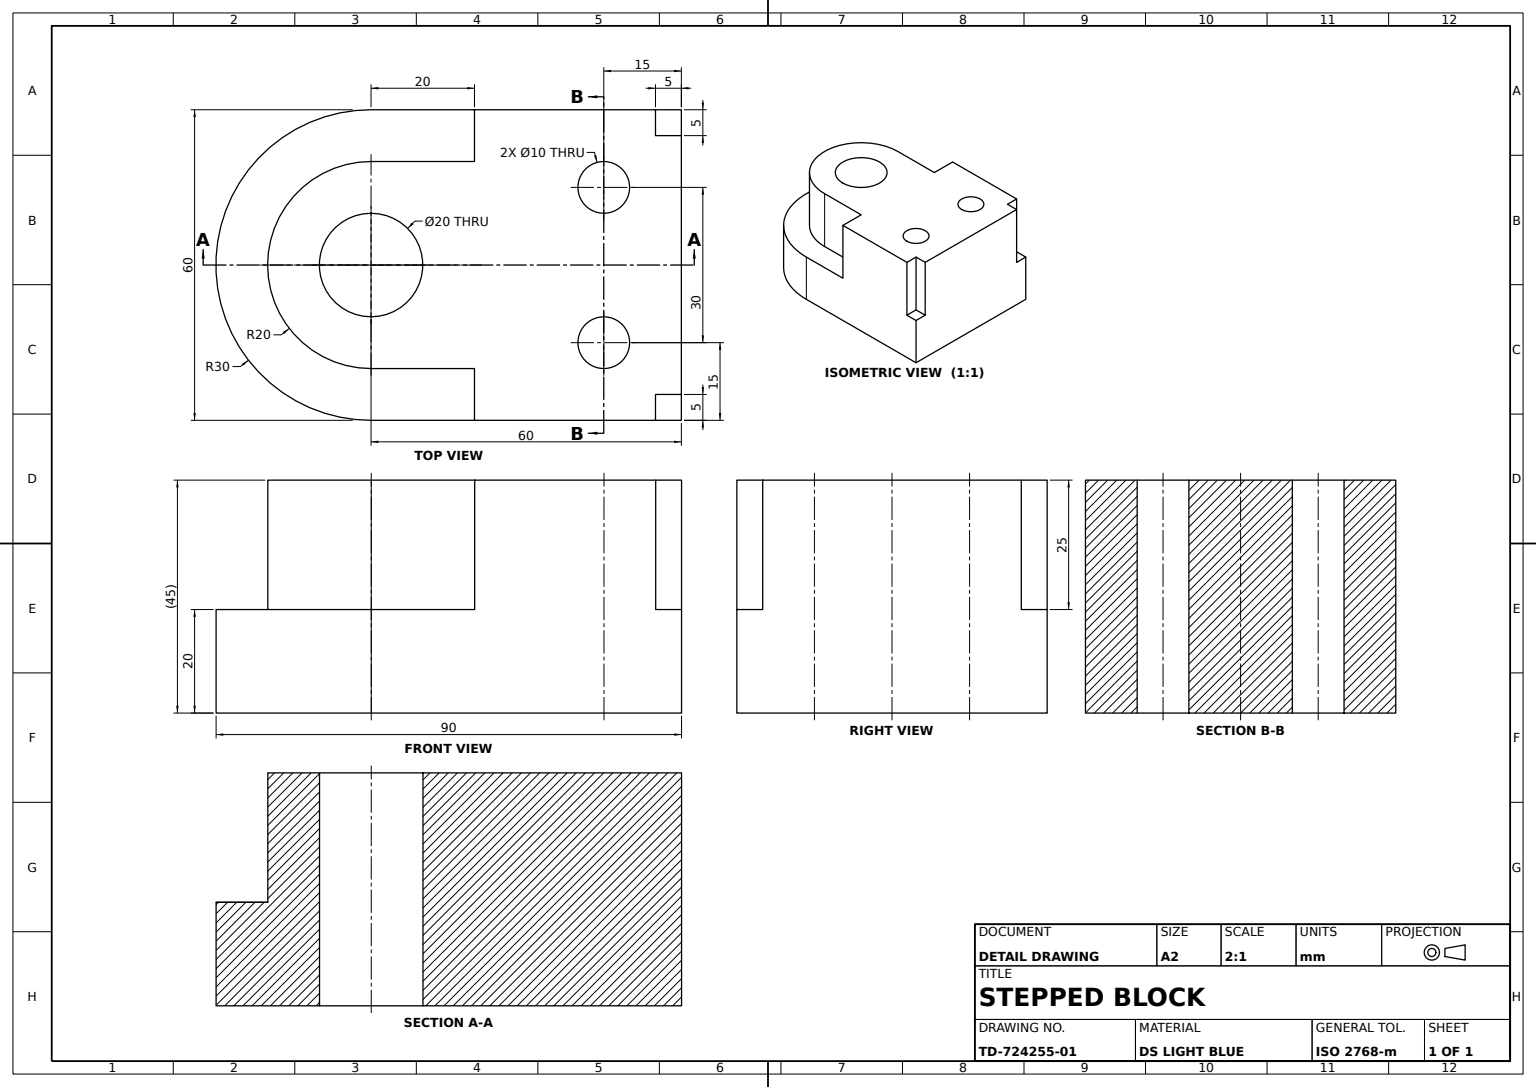
ISO-10303-21;
HEADER;
FILE_DESCRIPTION((''),'2;1');
FILE_NAME('','',(''),(''),'','','');
FILE_SCHEMA(('AUTOMOTIVE_DESIGN'));
ENDSEC;
DATA;
#1=APPLICATION_CONTEXT('');
#2=PRODUCT_CONTEXT('',#1,'mechanical');
#3=PRODUCT('','','',(#2));
#4=PRODUCT_DEFINITION_FORMATION('','',#3);
#5=PRODUCT_DEFINITION_CONTEXT('',#1,'design');
#6=PRODUCT_DEFINITION('','',#4,#5);
#7=PRODUCT_DEFINITION_SHAPE('','',#6);
#8=(LENGTH_UNIT()NAMED_UNIT(*)SI_UNIT(.MILLI.,.METRE.));
#9=(NAMED_UNIT(*)PLANE_ANGLE_UNIT()SI_UNIT($,.RADIAN.));
#10=(NAMED_UNIT(*)SI_UNIT($,.STERADIAN.)SOLID_ANGLE_UNIT());
#11=UNCERTAINTY_MEASURE_WITH_UNIT(LENGTH_MEASURE(0.005),#8,'distance_accuracy_value','');
#12=(GEOMETRIC_REPRESENTATION_CONTEXT(3)GLOBAL_UNCERTAINTY_ASSIGNED_CONTEXT((#11))GLOBAL_UNIT_ASSIGNED_CONTEXT((#8,#9,#10))REPRESENTATION_CONTEXT('',''));
#13=CARTESIAN_POINT('',(-30.,-30.,20.));
#14=VERTEX_POINT('',#13);
#15=CARTESIAN_POINT('',(30.,-30.,20.));
#16=VERTEX_POINT('',#15);
#17=CARTESIAN_POINT('',(0.,-30.,20.));
#18=DIRECTION('',(0.,0.,1.));
#19=DIRECTION('',(1.,0.,0.));
#20=AXIS2_PLACEMENT_3D('',#17,#18,#19);
#21=CIRCLE('',#20,30.);
#22=EDGE_CURVE('',#14,#16,#21,.T.);
#23=ORIENTED_EDGE('',*,*,#22,.F.);
#24=CARTESIAN_POINT('',(-30.,-30.,0.));
#25=VERTEX_POINT('',#24);
#26=CARTESIAN_POINT('',(-30.,-30.,10.));
#27=VECTOR('',#18,1000.);
#28=LINE('',#26,#27);
#29=EDGE_CURVE('',#25,#14,#28,.T.);
#30=ORIENTED_EDGE('',*,*,#29,.F.);
#31=CARTESIAN_POINT('',(30.,-30.,0.));
#32=VERTEX_POINT('',#31);
#33=CARTESIAN_POINT('',(0.,-30.,0.));
#34=AXIS2_PLACEMENT_3D('',#33,#18,#19);
#35=CIRCLE('',#34,30.);
#36=EDGE_CURVE('',#25,#32,#35,.T.);
#37=ORIENTED_EDGE('',*,*,#36,.T.);
#38=CARTESIAN_POINT('',(30.,-30.,10.));
#39=LINE('',#38,#27);
#40=EDGE_CURVE('',#32,#16,#39,.T.);
#41=ORIENTED_EDGE('',*,*,#40,.T.);
#42=EDGE_LOOP('',(#23,#30,#37,#41));
#43=FACE_BOUND('',#42,.T.);
#44=CARTESIAN_POINT('',(0.,-30.,10.));
#45=DIRECTION('',(0.,1.,0.));
#46=AXIS2_PLACEMENT_3D('',#44,#18,#45);
#47=CYLINDRICAL_SURFACE('',#46,30.);
#48=ADVANCED_FACE('',(#43),#47,.T.);
#49=CARTESIAN_POINT('',(20.,15.,45.));
#50=VERTEX_POINT('',#49);
#51=CARTESIAN_POINT('',(15.,15.,45.));
#52=AXIS2_PLACEMENT_3D('',#51,#18,#19);
#53=CIRCLE('',#52,5.);
#54=EDGE_CURVE('',#50,#50,#53,.T.);
#55=ORIENTED_EDGE('',*,*,#54,.T.);
#56=EDGE_LOOP('',(#55));
#57=FACE_BOUND('',#56,.T.);
#58=CARTESIAN_POINT('',(20.,15.,0.));
#59=VERTEX_POINT('',#58);
#60=CARTESIAN_POINT('',(15.,15.,0.));
#61=AXIS2_PLACEMENT_3D('',#60,#18,#19);
#62=CIRCLE('',#61,5.);
#63=EDGE_CURVE('',#59,#59,#62,.T.);
#64=ORIENTED_EDGE('',*,*,#63,.F.);
#65=EDGE_LOOP('',(#64));
#66=FACE_BOUND('',#65,.T.);
#67=CARTESIAN_POINT('',(15.,15.,21.84));
#68=AXIS2_PLACEMENT_3D('',#67,#18,#45);
#69=CYLINDRICAL_SURFACE('',#68,5.);
#70=ADVANCED_FACE('',(#57,#66),#69,.F.);
#71=CARTESIAN_POINT('',(-30.,-10.,20.));
#72=VERTEX_POINT('',#71);
#73=CARTESIAN_POINT('',(-30.,-10.,45.));
#74=VERTEX_POINT('',#73);
#75=CARTESIAN_POINT('',(-30.,-10.,0.));
#76=LINE('',#75,#27);
#77=EDGE_CURVE('',#72,#74,#76,.T.);
#78=ORIENTED_EDGE('',*,*,#77,.F.);
#79=CARTESIAN_POINT('',(-20.,-10.,20.));
#80=VERTEX_POINT('',#79);
#81=CARTESIAN_POINT('',(0.,-10.,20.));
#82=DIRECTION('',(-1.,0.,0.));
#83=VECTOR('',#82,1000.);
#84=LINE('',#81,#83);
#85=EDGE_CURVE('',#80,#72,#84,.T.);
#86=ORIENTED_EDGE('',*,*,#85,.F.);
#87=CARTESIAN_POINT('',(-20.,-10.,45.));
#88=VERTEX_POINT('',#87);
#89=LINE('',#79,#27);
#90=EDGE_CURVE('',#80,#88,#89,.T.);
#91=ORIENTED_EDGE('',*,*,#90,.T.);
#92=CARTESIAN_POINT('',(0.,-10.,45.));
#93=LINE('',#92,#83);
#94=EDGE_CURVE('',#88,#74,#93,.T.);
#95=ORIENTED_EDGE('',*,*,#94,.T.);
#96=EDGE_LOOP('',(#78,#86,#91,#95));
#97=FACE_BOUND('',#96,.T.);
#98=CARTESIAN_POINT('',(30.,-10.,20.));
#99=AXIS2_PLACEMENT_3D('',#98,#45,#82);
#100=PLANE('',#99);
#101=ADVANCED_FACE('',(#97),#100,.F.);
#102=CARTESIAN_POINT('',(-30.,30.,0.));
#103=VERTEX_POINT('',#102);
#104=CARTESIAN_POINT('',(30.,30.,0.));
#105=VERTEX_POINT('',#104);
#106=CARTESIAN_POINT('',(0.,30.,0.));
#107=VECTOR('',#19,1000.);
#108=LINE('',#106,#107);
#109=EDGE_CURVE('',#103,#105,#108,.T.);
#110=ORIENTED_EDGE('',*,*,#109,.T.);
#111=CARTESIAN_POINT('',(30.,0.,0.));
#112=DIRECTION('',(0.,-1.,0.));
#113=VECTOR('',#112,1000.);
#114=LINE('',#111,#113);
#115=EDGE_CURVE('',#105,#32,#114,.T.);
#116=ORIENTED_EDGE('',*,*,#115,.T.);
#117=ORIENTED_EDGE('',*,*,#36,.F.);
#118=CARTESIAN_POINT('',(-30.,0.,0.));
#119=VECTOR('',#45,1000.);
#120=LINE('',#118,#119);
#121=EDGE_CURVE('',#25,#103,#120,.T.);
#122=ORIENTED_EDGE('',*,*,#121,.T.);
#123=EDGE_LOOP('',(#110,#116,#117,#122));
#124=FACE_BOUND('',#123,.T.);
#125=ORIENTED_EDGE('',*,*,#63,.T.);
#126=EDGE_LOOP('',(#125));
#127=FACE_BOUND('',#126,.T.);
#128=CARTESIAN_POINT('',(-10.,15.,0.));
#129=VERTEX_POINT('',#128);
#130=CARTESIAN_POINT('',(-15.,15.,0.));
#131=AXIS2_PLACEMENT_3D('',#130,#18,#19);
#132=CIRCLE('',#131,5.);
#133=EDGE_CURVE('',#129,#129,#132,.T.);
#134=ORIENTED_EDGE('',*,*,#133,.T.);
#135=EDGE_LOOP('',(#134));
#136=FACE_BOUND('',#135,.T.);
#137=CARTESIAN_POINT('',(10.,-30.,0.));
#138=VERTEX_POINT('',#137);
#139=CIRCLE('',#34,10.);
#140=EDGE_CURVE('',#138,#138,#139,.T.);
#141=ORIENTED_EDGE('',*,*,#140,.T.);
#142=EDGE_LOOP('',(#141));
#143=FACE_BOUND('',#142,.T.);
#144=CARTESIAN_POINT('',(0.,0.,0.));
#145=AXIS2_PLACEMENT_3D('',#144,#18,#45);
#146=PLANE('',#145);
#147=ADVANCED_FACE('',(#124,#127,#136,#143),#146,.F.);
#148=CARTESIAN_POINT('',(25.,25.,20.));
#149=VERTEX_POINT('',#148);
#150=CARTESIAN_POINT('',(25.,25.,45.));
#151=VERTEX_POINT('',#150);
#152=LINE('',#148,#27);
#153=EDGE_CURVE('',#149,#151,#152,.T.);
#154=ORIENTED_EDGE('',*,*,#153,.T.);
#155=CARTESIAN_POINT('',(30.,25.,45.));
#156=VERTEX_POINT('',#155);
#157=CARTESIAN_POINT('',(-30.,25.,45.));
#158=LINE('',#157,#83);
#159=EDGE_CURVE('',#156,#151,#158,.T.);
#160=ORIENTED_EDGE('',*,*,#159,.F.);
#161=CARTESIAN_POINT('',(30.,25.,20.));
#162=VERTEX_POINT('',#161);
#163=CARTESIAN_POINT('',(30.,25.,0.));
#164=LINE('',#163,#27);
#165=EDGE_CURVE('',#162,#156,#164,.T.);
#166=ORIENTED_EDGE('',*,*,#165,.F.);
#167=CARTESIAN_POINT('',(-30.,25.,20.));
#168=LINE('',#167,#83);
#169=EDGE_CURVE('',#162,#149,#168,.T.);
#170=ORIENTED_EDGE('',*,*,#169,.T.);
#171=EDGE_LOOP('',(#154,#160,#166,#170));
#172=FACE_BOUND('',#171,.T.);
#173=AXIS2_PLACEMENT_3D('',#167,#112,#19);
#174=PLANE('',#173);
#175=ADVANCED_FACE('',(#172),#174,.F.);
#176=ORIENTED_EDGE('',*,*,#77,.T.);
#177=VERTEX_POINT('',#157);
#178=CARTESIAN_POINT('',(-30.,-30.,45.));
#179=LINE('',#178,#113);
#180=EDGE_CURVE('',#177,#74,#179,.T.);
#181=ORIENTED_EDGE('',*,*,#180,.F.);
#182=VERTEX_POINT('',#167);
#183=LINE('',#167,#27);
#184=EDGE_CURVE('',#182,#177,#183,.T.);
#185=ORIENTED_EDGE('',*,*,#184,.F.);
#186=CARTESIAN_POINT('',(-30.,30.,20.));
#187=VERTEX_POINT('',#186);
#188=CARTESIAN_POINT('',(-30.,0.,20.));
#189=LINE('',#188,#119);
#190=EDGE_CURVE('',#182,#187,#189,.T.);
#191=ORIENTED_EDGE('',*,*,#190,.T.);
#192=LINE('',#102,#27);
#193=EDGE_CURVE('',#103,#187,#192,.T.);
#194=ORIENTED_EDGE('',*,*,#193,.F.);
#195=ORIENTED_EDGE('',*,*,#121,.F.);
#196=ORIENTED_EDGE('',*,*,#29,.T.);
#197=EDGE_CURVE('',#14,#72,#189,.T.);
#198=ORIENTED_EDGE('',*,*,#197,.T.);
#199=EDGE_LOOP('',(#176,#181,#185,#191,#194,#195,#196,#198));
#200=FACE_BOUND('',#199,.T.);
#201=AXIS2_PLACEMENT_3D('',#24,#19,#45);
#202=PLANE('',#201);
#203=ADVANCED_FACE('',(#200),#202,.F.);
#204=ORIENTED_EDGE('',*,*,#133,.F.);
#205=EDGE_LOOP('',(#204));
#206=FACE_BOUND('',#205,.T.);
#207=CARTESIAN_POINT('',(-10.,15.,45.));
#208=VERTEX_POINT('',#207);
#209=CARTESIAN_POINT('',(-15.,15.,45.));
#210=AXIS2_PLACEMENT_3D('',#209,#18,#19);
#211=CIRCLE('',#210,5.);
#212=EDGE_CURVE('',#208,#208,#211,.T.);
#213=ORIENTED_EDGE('',*,*,#212,.T.);
#214=EDGE_LOOP('',(#213));
#215=FACE_BOUND('',#214,.T.);
#216=CARTESIAN_POINT('',(-15.,15.,21.84));
#217=AXIS2_PLACEMENT_3D('',#216,#18,#45);
#218=CYLINDRICAL_SURFACE('',#217,5.);
#219=ADVANCED_FACE('',(#206,#215),#218,.F.);
#220=ORIENTED_EDGE('',*,*,#212,.F.);
#221=EDGE_LOOP('',(#220));
#222=FACE_BOUND('',#221,.T.);
#223=ORIENTED_EDGE('',*,*,#54,.F.);
#224=EDGE_LOOP('',(#223));
#225=FACE_BOUND('',#224,.T.);
#226=CARTESIAN_POINT('',(30.,-10.,45.));
#227=VERTEX_POINT('',#226);
#228=CARTESIAN_POINT('',(30.,30.,45.));
#229=LINE('',#228,#119);
#230=EDGE_CURVE('',#227,#156,#229,.T.);
#231=ORIENTED_EDGE('',*,*,#230,.T.);
#232=ORIENTED_EDGE('',*,*,#159,.T.);
#233=CARTESIAN_POINT('',(25.,30.,45.));
#234=VERTEX_POINT('',#233);
#235=CARTESIAN_POINT('',(25.,0.,45.));
#236=LINE('',#235,#113);
#237=EDGE_CURVE('',#234,#151,#236,.T.);
#238=ORIENTED_EDGE('',*,*,#237,.F.);
#239=CARTESIAN_POINT('',(-25.,30.,45.));
#240=VERTEX_POINT('',#239);
#241=CARTESIAN_POINT('',(-30.,30.,45.));
#242=LINE('',#241,#83);
#243=EDGE_CURVE('',#234,#240,#242,.T.);
#244=ORIENTED_EDGE('',*,*,#243,.T.);
#245=CARTESIAN_POINT('',(-25.,25.,45.));
#246=VERTEX_POINT('',#245);
#247=CARTESIAN_POINT('',(-25.,0.,45.));
#248=LINE('',#247,#119);
#249=EDGE_CURVE('',#246,#240,#248,.T.);
#250=ORIENTED_EDGE('',*,*,#249,.F.);
#251=CARTESIAN_POINT('',(0.,25.,45.));
#252=LINE('',#251,#107);
#253=EDGE_CURVE('',#177,#246,#252,.T.);
#254=ORIENTED_EDGE('',*,*,#253,.F.);
#255=ORIENTED_EDGE('',*,*,#180,.T.);
#256=ORIENTED_EDGE('',*,*,#94,.F.);
#257=CARTESIAN_POINT('',(-20.,-30.,45.));
#258=VERTEX_POINT('',#257);
#259=CARTESIAN_POINT('',(-20.,0.,45.));
#260=LINE('',#259,#119);
#261=EDGE_CURVE('',#258,#88,#260,.T.);
#262=ORIENTED_EDGE('',*,*,#261,.F.);
#263=CARTESIAN_POINT('',(20.,-30.,45.));
#264=VERTEX_POINT('',#263);
#265=CARTESIAN_POINT('',(0.,-30.,45.));
#266=AXIS2_PLACEMENT_3D('',#265,#18,#19);
#267=CIRCLE('',#266,20.);
#268=EDGE_CURVE('',#258,#264,#267,.T.);
#269=ORIENTED_EDGE('',*,*,#268,.T.);
#270=CARTESIAN_POINT('',(20.,-10.,45.));
#271=VERTEX_POINT('',#270);
#272=CARTESIAN_POINT('',(20.,0.,45.));
#273=LINE('',#272,#113);
#274=EDGE_CURVE('',#271,#264,#273,.T.);
#275=ORIENTED_EDGE('',*,*,#274,.F.);
#276=EDGE_CURVE('',#227,#271,#93,.T.);
#277=ORIENTED_EDGE('',*,*,#276,.F.);
#278=EDGE_LOOP('',(#231,#232,#238,#244,#250,#254,#255,#256,#262,#269,#275,#277));
#279=FACE_BOUND('',#278,.T.);
#280=CARTESIAN_POINT('',(10.,-30.,45.));
#281=VERTEX_POINT('',#280);
#282=CIRCLE('',#266,10.);
#283=EDGE_CURVE('',#281,#281,#282,.T.);
#284=ORIENTED_EDGE('',*,*,#283,.F.);
#285=EDGE_LOOP('',(#284));
#286=FACE_BOUND('',#285,.T.);
#287=CARTESIAN_POINT('',(0.,0.,45.));
#288=AXIS2_PLACEMENT_3D('',#287,#18,#19);
#289=PLANE('',#288);
#290=ADVANCED_FACE('',(#222,#225,#279,#286),#289,.T.);
#291=ORIENTED_EDGE('',*,*,#140,.F.);
#292=EDGE_LOOP('',(#291));
#293=FACE_BOUND('',#292,.T.);
#294=ORIENTED_EDGE('',*,*,#283,.T.);
#295=EDGE_LOOP('',(#294));
#296=FACE_BOUND('',#295,.T.);
#297=CARTESIAN_POINT('',(0.,-30.,21.84));
#298=AXIS2_PLACEMENT_3D('',#297,#18,#45);
#299=CYLINDRICAL_SURFACE('',#298,10.);
#300=ADVANCED_FACE('',(#293,#296),#299,.F.);
#301=CARTESIAN_POINT('',(25.,30.,20.));
#302=VERTEX_POINT('',#301);
#303=CARTESIAN_POINT('',(25.,0.,20.));
#304=LINE('',#303,#113);
#305=EDGE_CURVE('',#302,#149,#304,.T.);
#306=ORIENTED_EDGE('',*,*,#305,.F.);
#307=LINE('',#301,#27);
#308=EDGE_CURVE('',#302,#234,#307,.T.);
#309=ORIENTED_EDGE('',*,*,#308,.T.);
#310=ORIENTED_EDGE('',*,*,#237,.T.);
#311=ORIENTED_EDGE('',*,*,#153,.F.);
#312=EDGE_LOOP('',(#306,#309,#310,#311));
#313=FACE_BOUND('',#312,.T.);
#314=AXIS2_PLACEMENT_3D('',#301,#82,#112);
#315=PLANE('',#314);
#316=ADVANCED_FACE('',(#313),#315,.F.);
#317=ORIENTED_EDGE('',*,*,#197,.F.);
#318=ORIENTED_EDGE('',*,*,#22,.T.);
#319=VERTEX_POINT('',#98);
#320=CARTESIAN_POINT('',(30.,0.,20.));
#321=LINE('',#320,#113);
#322=EDGE_CURVE('',#319,#16,#321,.T.);
#323=ORIENTED_EDGE('',*,*,#322,.F.);
#324=CARTESIAN_POINT('',(20.,-10.,20.));
#325=VERTEX_POINT('',#324);
#326=EDGE_CURVE('',#319,#325,#84,.T.);
#327=ORIENTED_EDGE('',*,*,#326,.T.);
#328=CARTESIAN_POINT('',(20.,-30.,20.));
#329=VERTEX_POINT('',#328);
#330=CARTESIAN_POINT('',(20.,0.,20.));
#331=LINE('',#330,#113);
#332=EDGE_CURVE('',#325,#329,#331,.T.);
#333=ORIENTED_EDGE('',*,*,#332,.T.);
#334=CARTESIAN_POINT('',(-20.,-30.,20.));
#335=VERTEX_POINT('',#334);
#336=CIRCLE('',#20,20.);
#337=EDGE_CURVE('',#335,#329,#336,.T.);
#338=ORIENTED_EDGE('',*,*,#337,.F.);
#339=CARTESIAN_POINT('',(-20.,0.,20.));
#340=LINE('',#339,#119);
#341=EDGE_CURVE('',#335,#80,#340,.T.);
#342=ORIENTED_EDGE('',*,*,#341,.T.);
#343=ORIENTED_EDGE('',*,*,#85,.T.);
#344=EDGE_LOOP('',(#317,#318,#323,#327,#333,#338,#342,#343));
#345=FACE_BOUND('',#344,.T.);
#346=CARTESIAN_POINT('',(0.,0.,20.));
#347=AXIS2_PLACEMENT_3D('',#346,#18,#45);
#348=PLANE('',#347);
#349=ADVANCED_FACE('',(#345),#348,.T.);
#350=LINE('',#324,#27);
#351=EDGE_CURVE('',#325,#271,#350,.T.);
#352=ORIENTED_EDGE('',*,*,#351,.F.);
#353=ORIENTED_EDGE('',*,*,#326,.F.);
#354=LINE('',#98,#27);
#355=EDGE_CURVE('',#319,#227,#354,.T.);
#356=ORIENTED_EDGE('',*,*,#355,.T.);
#357=ORIENTED_EDGE('',*,*,#276,.T.);
#358=EDGE_LOOP('',(#352,#353,#356,#357));
#359=FACE_BOUND('',#358,.T.);
#360=ADVANCED_FACE('',(#359),#100,.F.);
#361=ORIENTED_EDGE('',*,*,#355,.F.);
#362=ORIENTED_EDGE('',*,*,#322,.T.);
#363=ORIENTED_EDGE('',*,*,#40,.F.);
#364=ORIENTED_EDGE('',*,*,#115,.F.);
#365=CARTESIAN_POINT('',(30.,30.,20.));
#366=VERTEX_POINT('',#365);
#367=LINE('',#104,#27);
#368=EDGE_CURVE('',#105,#366,#367,.T.);
#369=ORIENTED_EDGE('',*,*,#368,.T.);
#370=EDGE_CURVE('',#366,#162,#321,.T.);
#371=ORIENTED_EDGE('',*,*,#370,.T.);
#372=ORIENTED_EDGE('',*,*,#165,.T.);
#373=ORIENTED_EDGE('',*,*,#230,.F.);
#374=EDGE_LOOP('',(#361,#362,#363,#364,#369,#371,#372,#373));
#375=FACE_BOUND('',#374,.T.);
#376=AXIS2_PLACEMENT_3D('',#104,#82,#112);
#377=PLANE('',#376);
#378=ADVANCED_FACE('',(#375),#377,.F.);
#379=CARTESIAN_POINT('',(-20.,-30.,32.5));
#380=LINE('',#379,#27);
#381=EDGE_CURVE('',#335,#258,#380,.T.);
#382=ORIENTED_EDGE('',*,*,#381,.T.);
#383=ORIENTED_EDGE('',*,*,#261,.T.);
#384=ORIENTED_EDGE('',*,*,#90,.F.);
#385=ORIENTED_EDGE('',*,*,#341,.F.);
#386=EDGE_LOOP('',(#382,#383,#384,#385));
#387=FACE_BOUND('',#386,.T.);
#388=AXIS2_PLACEMENT_3D('',#334,#19,#45);
#389=PLANE('',#388);
#390=ADVANCED_FACE('',(#387),#389,.F.);
#391=ORIENTED_EDGE('',*,*,#332,.F.);
#392=ORIENTED_EDGE('',*,*,#351,.T.);
#393=ORIENTED_EDGE('',*,*,#274,.T.);
#394=CARTESIAN_POINT('',(20.,-30.,32.5));
#395=LINE('',#394,#27);
#396=EDGE_CURVE('',#329,#264,#395,.T.);
#397=ORIENTED_EDGE('',*,*,#396,.F.);
#398=EDGE_LOOP('',(#391,#392,#393,#397));
#399=FACE_BOUND('',#398,.T.);
#400=AXIS2_PLACEMENT_3D('',#324,#82,#112);
#401=PLANE('',#400);
#402=ADVANCED_FACE('',(#399),#401,.F.);
#403=CARTESIAN_POINT('',(0.,30.,20.));
#404=LINE('',#403,#107);
#405=EDGE_CURVE('',#302,#366,#404,.T.);
#406=ORIENTED_EDGE('',*,*,#405,.F.);
#407=ORIENTED_EDGE('',*,*,#305,.T.);
#408=ORIENTED_EDGE('',*,*,#169,.F.);
#409=ORIENTED_EDGE('',*,*,#370,.F.);
#410=EDGE_LOOP('',(#406,#407,#408,#409));
#411=FACE_BOUND('',#410,.T.);
#412=ADVANCED_FACE('',(#411),#348,.T.);
#413=CARTESIAN_POINT('',(-25.,25.,20.));
#414=VERTEX_POINT('',#413);
#415=LINE('',#413,#27);
#416=EDGE_CURVE('',#414,#246,#415,.T.);
#417=ORIENTED_EDGE('',*,*,#416,.F.);
#418=CARTESIAN_POINT('',(0.,25.,20.));
#419=LINE('',#418,#107);
#420=EDGE_CURVE('',#182,#414,#419,.T.);
#421=ORIENTED_EDGE('',*,*,#420,.F.);
#422=ORIENTED_EDGE('',*,*,#184,.T.);
#423=ORIENTED_EDGE('',*,*,#253,.T.);
#424=EDGE_LOOP('',(#417,#421,#422,#423));
#425=FACE_BOUND('',#424,.T.);
#426=ADVANCED_FACE('',(#425),#174,.F.);
#427=ORIENTED_EDGE('',*,*,#337,.T.);
#428=ORIENTED_EDGE('',*,*,#396,.T.);
#429=ORIENTED_EDGE('',*,*,#268,.F.);
#430=ORIENTED_EDGE('',*,*,#381,.F.);
#431=EDGE_LOOP('',(#427,#428,#429,#430));
#432=FACE_BOUND('',#431,.T.);
#433=CARTESIAN_POINT('',(0.,-30.,32.5));
#434=AXIS2_PLACEMENT_3D('',#433,#18,#19);
#435=CYLINDRICAL_SURFACE('',#434,20.);
#436=ADVANCED_FACE('',(#432),#435,.T.);
#437=ORIENTED_EDGE('',*,*,#416,.T.);
#438=ORIENTED_EDGE('',*,*,#249,.T.);
#439=CARTESIAN_POINT('',(-25.,30.,20.));
#440=VERTEX_POINT('',#439);
#441=CARTESIAN_POINT('',(-25.,30.,0.));
#442=LINE('',#441,#27);
#443=EDGE_CURVE('',#440,#240,#442,.T.);
#444=ORIENTED_EDGE('',*,*,#443,.F.);
#445=CARTESIAN_POINT('',(-25.,0.,20.));
#446=LINE('',#445,#119);
#447=EDGE_CURVE('',#414,#440,#446,.T.);
#448=ORIENTED_EDGE('',*,*,#447,.F.);
#449=EDGE_LOOP('',(#437,#438,#444,#448));
#450=FACE_BOUND('',#449,.T.);
#451=AXIS2_PLACEMENT_3D('',#413,#19,#45);
#452=PLANE('',#451);
#453=ADVANCED_FACE('',(#450),#452,.F.);
#454=ORIENTED_EDGE('',*,*,#368,.F.);
#455=ORIENTED_EDGE('',*,*,#109,.F.);
#456=ORIENTED_EDGE('',*,*,#193,.T.);
#457=EDGE_CURVE('',#187,#440,#404,.T.);
#458=ORIENTED_EDGE('',*,*,#457,.T.);
#459=ORIENTED_EDGE('',*,*,#443,.T.);
#460=ORIENTED_EDGE('',*,*,#243,.F.);
#461=ORIENTED_EDGE('',*,*,#308,.F.);
#462=ORIENTED_EDGE('',*,*,#405,.T.);
#463=EDGE_LOOP('',(#454,#455,#456,#458,#459,#460,#461,#462));
#464=FACE_BOUND('',#463,.T.);
#465=AXIS2_PLACEMENT_3D('',#102,#112,#19);
#466=PLANE('',#465);
#467=ADVANCED_FACE('',(#464),#466,.F.);
#468=ORIENTED_EDGE('',*,*,#447,.T.);
#469=ORIENTED_EDGE('',*,*,#457,.F.);
#470=ORIENTED_EDGE('',*,*,#190,.F.);
#471=ORIENTED_EDGE('',*,*,#420,.T.);
#472=EDGE_LOOP('',(#468,#469,#470,#471));
#473=FACE_BOUND('',#472,.T.);
#474=ADVANCED_FACE('',(#473),#348,.T.);
#475=CLOSED_SHELL('',(#48,#70,#101,#147,#175,#203,#219,#290,#300,#316,#349,#360,#378,#390,#402,#412,#426,#436,#453,#467,#474));
#476=MANIFOLD_SOLID_BREP('',#475);
#477=ADVANCED_BREP_SHAPE_REPRESENTATION('',(#476),#12);
#478=SHAPE_DEFINITION_REPRESENTATION(#7,#477);
ENDSEC;
END-ISO-10303-21;
